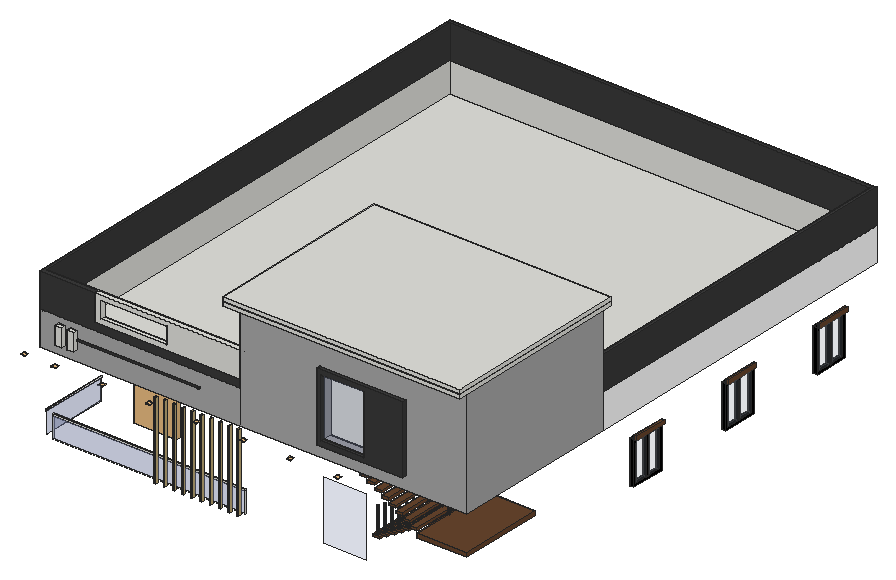
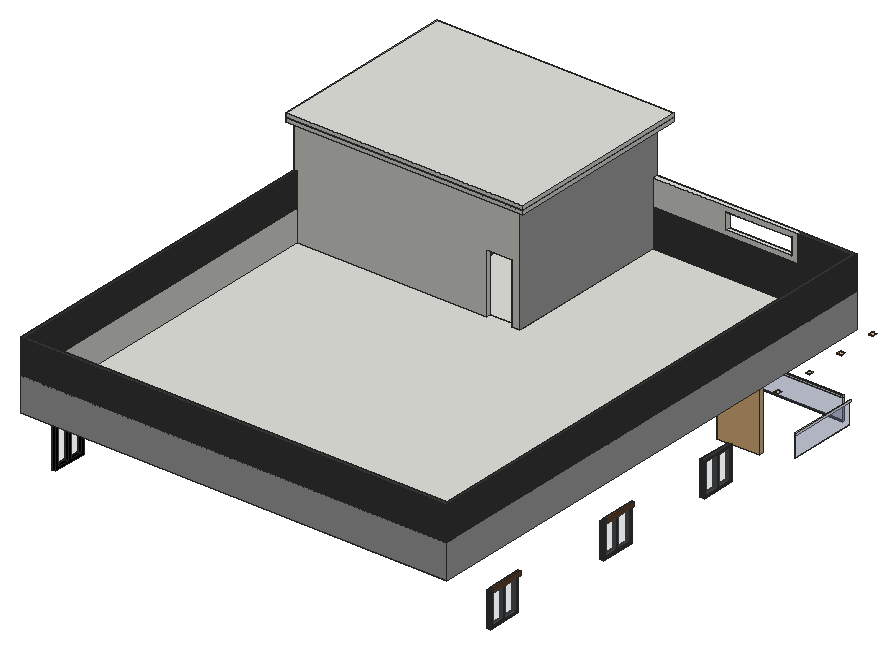
# SketchUp Ruby script. Lengths in inches.
U = 1.inch
M = Sketchup.active_model
def pt(a) = Geom::Point3d.new(a.map { |v| v * U })
def face(e, loops, mat)
  f = e.add_face(loops[0].map { |a| pt(a) })
  loops[1..].each { |l| e.add_face(l.map { |a| pt(a) }).erase! }
  f.material = f.back_material = mat if mat
  f
end
# faces: each face lists its corners as indices into pts; further lists are holes
def faces(e, pts, list, mat = nil) = list.each { |f| face(e, (f[0].is_a?(Array) ? f : [f]).map { |l| l.map { |i| pts[i] } }, mat) }
# xy, xz, yz: faces in a plane at the given z, y or x. An outline is a flat list of corners, or four numbers for a rectangle; further outlines are holes
def ring(l) = l.size == 4 ? [[l[0], l[1]], [l[2], l[1]], [l[2], l[3]], [l[0], l[3]]] : l.each_slice(2).to_a
def flat(e, list, mat, &to3) = list.each { |f| face(e, (f[0].is_a?(Array) ? f : [f]).map { |l| ring(l).map { |u, v| to3.(u, v) } }, mat) }
def xy(e, z, list, mat = nil) = flat(e, list, mat) { |x, y| [x, y, z] }
def xz(e, y, list, mat = nil) = flat(e, list, mat) { |x, z| [x, y, z] }
def yz(e, x, list, mat = nil) = flat(e, list, mat) { |y, z| [x, y, z] }
def lines(e, pts, list) = list.each { |a, b| e.add_line(pt(pts[a]), pt(pts[b])) }
# prism: a flat outline (further loops are holes) pulled along v
def prism(e, loops, v, mat = nil)
  f = face(e, loops, mat); d = Geom::Vector3d.new(v.map { |x| x * U })
  f.pushpull(f.normal.samedirection?(d) ? d.length : -d.length)
end
def box(e, o, s, mat = nil) = prism(e, [[o, [o[0] + s[0], o[1], o[2]], [o[0] + s[0], o[1] + s[1], o[2]], [o[0], o[1] + s[1], o[2]]]], [0, 0, s[2]], mat)
def at(x, y, z, deg = 0) = Geom::Transformation.translation(pt([x, y, z])) * Geom::Transformation.rotation(ORIGIN, Z_AXIS, deg.degrees)
def axes(o, x, y, z) = Geom::Transformation.new([*x, 0, *y, 0, *z, 0, *pt(o).to_a, 1])
def part(name) = M.definitions.add(name)
# library, detail: a bought-in or finely detailed component or shape, given as its bounding box
def library(name, o, s) = part(name).tap { |d| box(d.entities, o, s) }
def detail(e, o, s) = box(e.add_group.entities, o, s)
def put(e, d, t, mat = nil) = e.add_instance(d, t).tap { |i| i.material = mat if mat }
def group(e, t, mat = nil) = e.add_group.tap { |g| g.transformation = t; g.material = mat if mat }.entities
root = M.entities
M.materials.add("Glass_Basic_01").color = [161, 173, 186]
M.materials["Glass_Basic_01"].alpha = 0.25
M.materials.add("Glass_Sky Reflection_01").color = [126, 138, 183]
M.materials["Glass_Sky Reflection_01"].alpha = 0.25
M.materials.add("M00_Soft_Cloud").color = [255, 255, 255]
M.materials.add("M03_Pewter_Shine").color = [168, 168, 168]
M.materials.add("M07_Charcoal_Gleam").color = [58, 58, 58]
M.materials.add("M09_Shadow_Night").color = [0, 0, 0]
M.materials.add("Metal_06_1K").color = [238, 236, 231]
M.materials.add("Metal_10_1K").color = [196, 175, 123]
M.materials.add("Wood_Veneer_15_1K").color = [103, 69, 45]
c1 = part("Stair tread")
xy(c1.entities,3,[[0,0,10,60]],"Wood_Veneer_15_1K")
xy(c1.entities,6,[[0,0,10,60]],"Wood_Veneer_15_1K")
xz(c1.entities,0,[[0,3,10,6]],"Wood_Veneer_15_1K")
xz(c1.entities,60,[[0,3,10,6]])
yz(c1.entities,0,[[0,3,60,6]],"Wood_Veneer_15_1K")
yz(c1.entities,10,[[0,3,60,6]],"Wood_Veneer_15_1K")
c2 = part("Tread with baluster")
box(c2.entities,[0,0,3],[10,60,3])
g1 = group(c2.entities,at(3.7,1.6875,6))
prism(g1,[[[0.9375,0,0],[0.69,0.03,0],[0.47,0.125,0],[0.27,0.27,0],[0.125,0.47,0],[0.03,0.69,0],[0,0.9375,0],[0.03,1.18,0],[0.125,1.41,0],[0.27,1.6,0],[0.47,1.75,0],[0.69,1.84,0],[0.9375,1.875,0],[1.18,1.84,0],[1.41,1.75,0],[1.6,1.6,0],[1.75,1.41,0],[1.84,1.18,0],[1.875,0.9375,0],[1.84,0.69,0],[1.75,0.47,0],[1.6,0.27,0],[1.41,0.125,0],[1.18,0.03,0]]],[0,0,36.125],"Metal_06_1K")
c3 = part("Group\#49")
put(c3.entities,c1,at(70,0,87))
put(c3.entities,c1,at(60,0,93))
put(c3.entities,c1,at(30,0,111))
put(c3.entities,c1,at(90,0,75))
put(c3.entities,c1,at(10,0,123))
put(c3.entities,c1,at(20,0,117))
put(c3.entities,c1,at(50,0,99))
put(c3.entities,c1,at(40,0,105))
put(c3.entities,c1,at(100,0,69))
put(c3.entities,c1,at(80,0,81))
put(c3.entities,c2,at(100,60,57),"Wood_Veneer_15_1K")
put(c3.entities,c2,at(40,60,21),"Wood_Veneer_15_1K")
put(c3.entities,c2,at(60,60,33),"Wood_Veneer_15_1K")
put(c3.entities,c2,at(80,60,45),"Wood_Veneer_15_1K")
put(c3.entities,c2,at(90,60,51),"Wood_Veneer_15_1K")
put(c3.entities,c2,at(70,60,39),"Wood_Veneer_15_1K")
put(c3.entities,c2,at(10,60,3),"Wood_Veneer_15_1K")
put(c3.entities,c2,at(50,60,27),"Wood_Veneer_15_1K")
put(c3.entities,c2,at(30,60,15),"Wood_Veneer_15_1K")
put(c3.entities,c2,at(0,60,-3),"Wood_Veneer_15_1K")
put(c3.entities,c2,at(20,60,9),"Wood_Veneer_15_1K")
g2 = group(c3.entities,at(110,60,63),"Wood_Veneer_15_1K")
box(g2,[0,-60,0],[70,120,6])
c4 = library("Group\#33",[0,0,0],[60,6,84])
c5 = part("Group\#14")
box(c5.entities,[0,0,0],[2.5,2.9375,108.625],"Metal_10_1K")
c6 = part("Group\#41")
xz(c6.entities,0,[[0,0,60,84]],"Glass_Sky Reflection_01")
c7 = part("Group\#23")
xy(c7.entities,0,[[-6,0,0,48]],"M07_Charcoal_Gleam")
xy(c7.entities,3,[[-6,3,0,23],[-6,25,0,45]],"M07_Charcoal_Gleam")
xy(c7.entities,45,[[-6,3,0,23],[-6,25,0,45]],"M07_Charcoal_Gleam")
xy(c7.entities,48,[[-6,0,0,48]],"M07_Charcoal_Gleam")
xz(c7.entities,0,[[-6,0,0,48]],"M07_Charcoal_Gleam")
xz(c7.entities,3,[[-6,3,0,45]],"M07_Charcoal_Gleam")
xz(c7.entities,23,[[-6,3,0,45]],"M07_Charcoal_Gleam")
xz(c7.entities,25,[[-6,3,0,45]],"M07_Charcoal_Gleam")
xz(c7.entities,45,[[-6,3,0,45]],"M07_Charcoal_Gleam")
xz(c7.entities,48,[[-6,0,0,48]],"M07_Charcoal_Gleam")
yz(c7.entities,-6,[[3,3,23,45],[25,3,45,45]],"Glass_Basic_01")
yz(c7.entities,-6,[[[0,0,48,48],[3,3,45,45]],[23,3,25,45]],"M07_Charcoal_Gleam")
yz(c7.entities,0,[[[0,0,48,48],[25,3,45,45],[3,3,23,45]]],"M07_Charcoal_Gleam")
c8 = part("Group\#21")
xy(c8.entities,0,[[0,0,6,48]],"M09_Shadow_Night")
xy(c8.entities,3,[[0,3,6,23],[0,25,6,45]],"M09_Shadow_Night")
xy(c8.entities,56.625,[[0,3,6,23],[0,25,6,45]],"M09_Shadow_Night")
xy(c8.entities,59.625,[[0,0,6,48]],"M09_Shadow_Night")
xz(c8.entities,0,[[0,0,6,59.625]],"M09_Shadow_Night")
xz(c8.entities,3,[[0,3,6,56.625]],"M09_Shadow_Night")
xz(c8.entities,23,[[0,3,6,56.625]],"M09_Shadow_Night")
xz(c8.entities,25,[[0,3,6,56.625]],"M09_Shadow_Night")
xz(c8.entities,45,[[0,3,6,56.625]],"M09_Shadow_Night")
xz(c8.entities,48,[[0,0,6,59.625]],"M09_Shadow_Night")
yz(c8.entities,0,[[[0,0,48,59.625],[25,3,45,56.625],[3,3,23,56.625]]],"M09_Shadow_Night")
yz(c8.entities,6,[[3,3,23,56.625],[25,3,45,56.625]],"Glass_Basic_01")
yz(c8.entities,6,[[[0,0,48,59.625],[3,3,45,56.625]],[23,3,25,56.625]],"M09_Shadow_Night")
c9 = part("Group\#22")
box(c9.entities,[-4,0,0],[4,48,6],"Wood_Veneer_15_1K")
c10 = part("Group\#20")
box(c10.entities,[-4,0,0],[4,48,6],"Wood_Veneer_15_1K")
c11 = part("Group\#35")
detail(c11.entities,[0,0,-0.5],[5.96,5.96,0.5])
put(root,c3,at(9361.9375,4417.5625,155.625))
put(root,c4,at(8998.12,4512.1,155.625))
g3 = group(root,at(9232.37,4414.5625,165.625))
xy(g3,0,[[-269.43,0,0,0.9375]])
xy(g3,30,[[-269.43,-1,0,0],[-269.43,0,0,0.9375]])
xy(g3,32,[[-269.43,-1,0,0.9375]])
xz(g3,-1,[[-269.43,30,0,32]])
xz(g3,0,[[-269.43,0,0,30]],"Glass_Sky Reflection_01")
xz(g3,0.9375,[[-269.43,30,0,32]])
xz(g3,0.9375,[[-269.43,0,0,30]],"Glass_Sky Reflection_01")
yz(g3,-269.43,[[0,0,0.9375,30],[-1,30,0.9375,32]])
yz(g3,0,[[0,0,0.9375,30],[-1,30,0.9375,32]])
g4 = group(g3,at(-281.43,3,0),"Glass_Sky Reflection_01")
xy(g4,0,[[0,0,0.95,96]])
xy(g4,30,[[0,0,0.95,96]])
xy(g4,30,[[-1,0,0,96]],"M00_Soft_Cloud")
xy(g4,32,[[-1,0,0.95,96]],"M00_Soft_Cloud")
xz(g4,0,[[0,0,0.95,30]])
xz(g4,0,[[-1,30,0.95,32]],"M00_Soft_Cloud")
xz(g4,96,[[0,0,0.95,30],[-1,30,0.95,32]])
yz(g4,-1,[[0,30,96,32]],"M00_Soft_Cloud")
yz(g4,0,[[0,0,96,30]])
yz(g4,0.95,[[0,0,96,30]],"Glass_Sky Reflection_01")
yz(g4,0.95,[[0,30,96,32]],"M00_Soft_Cloud")
put(root,c5,at(9227.55,4406.82,165.625))
put(root,c5,at(9214.6,4406.82,165.625))
put(root,c5,at(9201.65,4406.82,165.625))
put(root,c5,at(9188.7,4406.82,165.625))
put(root,c5,at(9175.75,4406.82,165.625))
put(root,c5,at(9162.8,4406.82,165.625))
put(root,c5,at(9149.85,4406.82,165.625))
put(root,c5,at(9136.9,4406.82,165.625))
put(root,c5,at(9123.94,4406.82,165.625))
put(root,c5,at(9110.99,4406.82,165.625))
put(root,c6,at(9351.1,4404.65,174))
put(root,c7,at(8956.9375,5000.875,185.625))
put(root,c7,at(8956.9375,4802.0625,185.625))
put(root,c7,at(8956.9375,4625.6875,185.625))
put(root,c8,at(9544.9375,4700.125,186))
put(root,c8,at(9544.9375,4861.625,186))
put(root,c8,at(9544.9375,5022.125,186))
put(root,c9,at(8950.9375,5000.875,233.625))
put(root,c9,at(8950.9375,4802.0625,233.625))
put(root,c9,at(9554.9375,4700.125,245.625))
put(root,c10,at(9554.9375,4861.625,245.625))
put(root,c10,at(9554.9375,5022.125,245.625))
put(root,c11,at(8979.85,4389.8,274.25))
put(root,c11,at(9046.04,4389.8,274.25))
put(root,c11,at(9112.22,4389.8,274.25))
put(root,c11,at(9178.41,4389.8,274.25))
put(root,c11,at(9244.6,4389.8,274.25))
put(root,c11,at(9310.79,4389.8,274.25))
put(root,c11,at(9376.97,4389.8,274.25))
put(root,c11,at(8936.47,4389.8,274.25))
put(root,c11,at(8936.47,4445.26,274.25))
put(root,c11,at(8936.47,4500.72,274.25))
put(root,c11,at(8936.47,4556.18,274.25))
g5 = group(root,at(8950.9375,4405.5625,281.25))
xy(g5,0,[[0,0,600,720]])
xy(g5,6,[[5,6.8125,281.43,6.8125,281.43,240,292.55,240,292.55,234,328.55,234,328.55,240,595,240,595,715,5,715],[281.43,6.8125,287.43,234],[287.43,12,591,234],[281.43,234,292.55,240],[328.55,234,591,240]])
xy(g5,24.375,[[400.16,0,460.16,12]],"M03_Pewter_Shine")
xy(g5,47.625,[[0,0,5,715],[595,240,600,720],[0,715,595,720]])
xy(g5,58.75,[[77.52,0,281.43,6.8125]])
xy(g5,65.38,[[85.88,0,178.94,6.8125]])
xy(g5,88.82,[[85.88,0,178.94,6.8125]])
xy(g5,90,[[292.55,234,328.55,240]])
xy(g5,95.625,[[77.52,0,281.43,6.8125]])
xy(g5,95.625,[[0,0,77.52,0,77.52,6.8125,5,6.8125,5,715,0,715],[595,240,600,720],[0,715,595,720]],"M07_Charcoal_Gleam")
xy(g5,108.375,[[400.16,0,460.16,12]],"M03_Pewter_Shine")
xy(g5,156,[[[281.43,0,600,240],[287.43,12,591,234]]])
xz(g5,0,[[[77.52,58.75,281.43,95.625],[85.88,65.38,178.94,88.82]]])
xz(g5,0,[[0,0,281.43,47.625],[[281.43,0,600,156],[400.16,24.375,460.16,108.375]]],"M03_Pewter_Shine")
xz(g5,0,[[0,47.625,281.43,47.625,281.43,58.75,77.52,58.75,77.52,95.625,0,95.625]],"M07_Charcoal_Gleam")
xz(g5,6.8125,[[281.43,6,287.43,27.625],[281.43,27.625,287.43,47.625],[281.43,47.625,287.43,58.75],[[77.52,58.75,281.43,95.625],[85.88,65.38,178.94,88.82]],[281.43,58.75,287.43,95.625]])
xz(g5,6.8125,[[5,6,5,95.625,77.52,95.625,77.52,58.75,281.43,58.75,281.43,6]],"M07_Charcoal_Gleam")
xz(g5,12,[[[287.43,6,591,156],[400.16,24.375,460.16,108.375]]],"M03_Pewter_Shine")
xz(g5,234,[[287.43,6,292.55,6,292.55,90,328.55,90,328.55,6,591,6,591,156,287.43,156]],"M03_Pewter_Shine")
xz(g5,240,[[281.43,6,281.43,156,600,156,600,95.625,595,95.625,595,6,328.55,6,328.55,90,292.55,90,292.55,6]])
xz(g5,715,[[5,6,595,47.625],[0,47.625,5,95.625]])
xz(g5,715,[[5,47.625,595,95.625]],"M07_Charcoal_Gleam")
xz(g5,720,[[0,0,600,47.625]],"M03_Pewter_Shine")
xz(g5,720,[[0,47.625,595,95.625],[595,47.625,600,95.625]],"M07_Charcoal_Gleam")
yz(g5,0,[[0,0,720,47.625]],"M03_Pewter_Shine")
yz(g5,0,[[0,47.625,715,95.625],[715,47.625,720,95.625]],"M07_Charcoal_Gleam")
yz(g5,5,[[6.8125,6,715,47.625]])
yz(g5,5,[[6.8125,47.625,715,95.625]],"M07_Charcoal_Gleam")
yz(g5,77.52,[[0,58.75,6.8125,95.625]])
yz(g5,85.88,[[0,65.38,6.8125,88.82]])
yz(g5,178.94,[[0,65.38,6.8125,88.82]])
yz(g5,281.43,[[0,47.625,6.8125,58.75],[0,58.75,6.8125,95.625]])
yz(g5,281.43,[[6.8125,6,6.8125,95.625,0,95.625,0,156,240,156,240,6]],"M03_Pewter_Shine")
yz(g5,287.43,[[12,6,234,156]],"M03_Pewter_Shine")
yz(g5,292.55,[[234,6,240,90]])
yz(g5,328.55,[[234,6,240,90]])
yz(g5,400.16,[[0,24.375,12,108.375]],"M03_Pewter_Shine")
yz(g5,460.16,[[0,24.375,12,108.375]],"M03_Pewter_Shine")
yz(g5,591,[[12,6,234,156]],"M03_Pewter_Shine")
yz(g5,595,[[240,6,715,47.625],[234,47.625,240,95.625],[715,47.625,720,95.625]])
yz(g5,595,[[240,47.625,715,95.625]],"M07_Charcoal_Gleam")
yz(g5,600,[[240,0,720,47.625]],"M00_Soft_Cloud")
yz(g5,600,[[0,0,240,156]],"M03_Pewter_Shine")
yz(g5,600,[[240,47.625,720,95.625]],"M07_Charcoal_Gleam")
p = [[60.5,6.8125,27.625],[60.5,0,27.625],[287.43,6.8125,95.625],[287.43,0,95.625],[591,234,47.625],[595,234,47.625]]
lines(g5,p,[[0,1],[2,3],[4,5]])
put(root,c3,at(9361.9375,4417.5625,287.25))
g6 = group(root,at(8974.94,4405.5625,295.49))
box(g6,[2.75,-6,0],[9.125,6,24.875])
g7 = group(root,at(8991.5,4405.5625,295.49))
box(g7,[2.75,-6,0],[9.125,6,24.875])
g8 = group(root,at(9351.1,4405.5625,305.625))
prism(g8,[[[-6,0,-6],[-6,0,90],[114.5,0,90],[114.5,0,-6]],[[60,0,84],[0,0,84],[0,0,0],[60,0,0]]],[0,-6,0],"M07_Charcoal_Gleam")
put(root,c6,at(9351.1,4405.5625,305.625))
g9 = group(root,at(9003.38,4405.5625,307.92))
box(g9,[0,-1,0],[173.32,1,2.84],"M07_Charcoal_Gleam")
g10 = group(root,at(9232.37,4405.5625,437.25))
xy(g10,0,[[-8,-20,324.57,246]])
xy(g10,5,[[-3,-3,321.57,243]])
xy(g10,5,[[-8,-20,324.57,-3],[-8,-3,-3,246],[321.57,-3,324.57,246],[-3,243,321.57,246]],"M09_Shadow_Night")
xy(g10,7,[[-3,-3,321.57,243]])
xy(g10,7,[[-8,-20,324.57,-3],[-8,-3,-3,246],[321.57,-3,324.57,246],[-3,243,321.57,246]],"M09_Shadow_Night")
xy(g10,12,[[-8,-20,324.57,246]])
xz(g10,-20,[[-8,0,324.57,5],[-8,7,324.57,12]])
xz(g10,-3,[[-3,5,321.57,7]],"M09_Shadow_Night")
xz(g10,243,[[-3,5,321.57,7]],"M09_Shadow_Night")
xz(g10,246,[[-8,0,324.57,5],[-8,7,324.57,12]])
yz(g10,-8,[[-20,0,246,5],[-20,7,246,12]])
yz(g10,-3,[[-3,5,243,7]],"M09_Shadow_Night")
yz(g10,321.57,[[-3,5,243,7]],"M09_Shadow_Night")
yz(g10,324.57,[[-20,0,246,5],[-20,7,246,12]])
